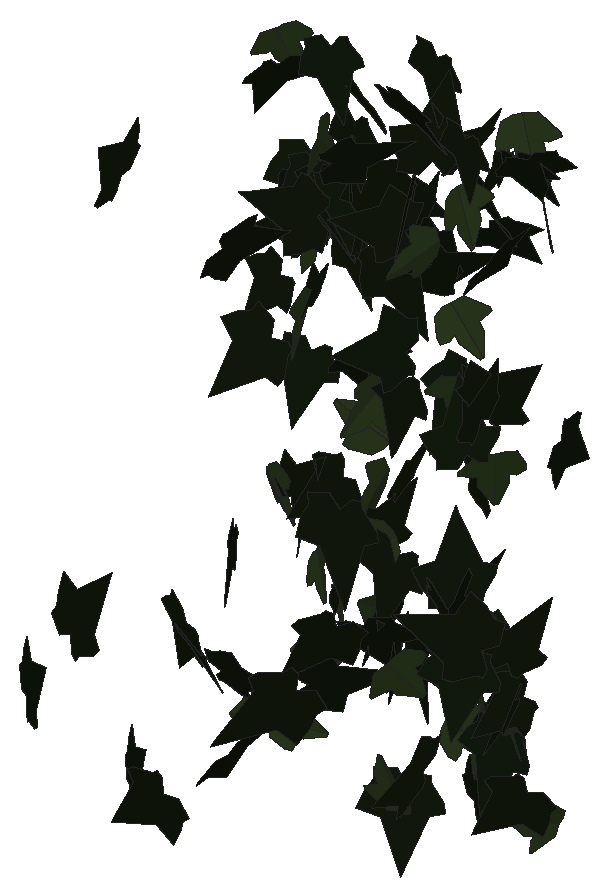
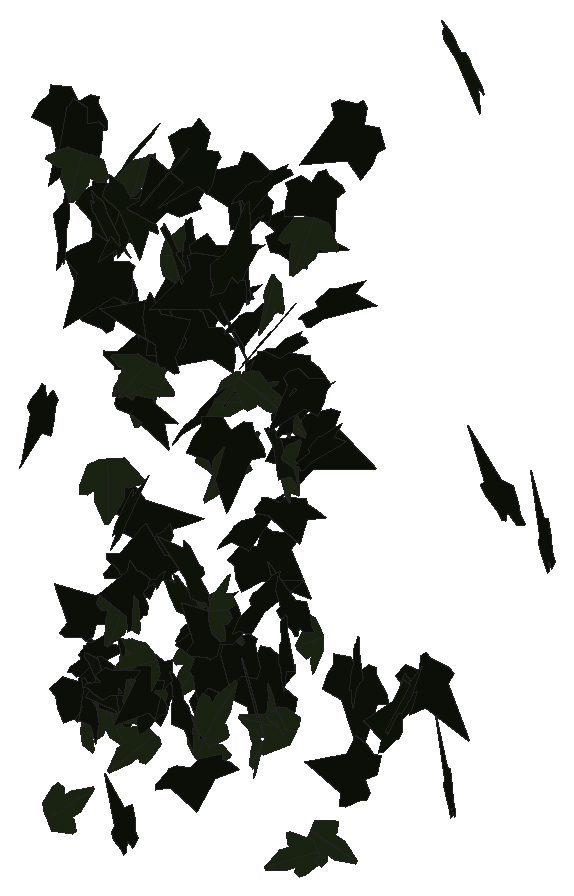
# SketchUp Ruby script. Lengths in inches.
U = 1.inch
M = Sketchup.active_model
def pt(a) = Geom::Point3d.new(a.map { |v| v * U })
def face(e, loops, mat)
  f = e.add_face(loops[0].map { |a| pt(a) })
  loops[1..].each { |l| e.add_face(l.map { |a| pt(a) }).erase! }
  f.material = f.back_material = mat if mat
  f
end
# faces: each face lists its corners as indices into pts; further lists are holes
def faces(e, pts, list, mat = nil) = list.each { |f| face(e, (f[0].is_a?(Array) ? f : [f]).map { |l| l.map { |i| pts[i] } }, mat) }
# xy, xz, yz: faces in a plane at the given z, y or x. An outline is a flat list of corners, or four numbers for a rectangle; further outlines are holes
def ring(l) = l.size == 4 ? [[l[0], l[1]], [l[2], l[1]], [l[2], l[3]], [l[0], l[3]]] : l.each_slice(2).to_a
def flat(e, list, mat, &to3) = list.each { |f| face(e, (f[0].is_a?(Array) ? f : [f]).map { |l| ring(l).map { |u, v| to3.(u, v) } }, mat) }
def xy(e, z, list, mat = nil) = flat(e, list, mat) { |x, y| [x, y, z] }
def xz(e, y, list, mat = nil) = flat(e, list, mat) { |x, z| [x, y, z] }
def yz(e, x, list, mat = nil) = flat(e, list, mat) { |y, z| [x, y, z] }
def lines(e, pts, list) = list.each { |a, b| e.add_line(pt(pts[a]), pt(pts[b])) }
# prism: a flat outline (further loops are holes) pulled along v
def prism(e, loops, v, mat = nil)
  f = face(e, loops, mat); d = Geom::Vector3d.new(v.map { |x| x * U })
  f.pushpull(f.normal.samedirection?(d) ? d.length : -d.length)
end
def box(e, o, s, mat = nil) = prism(e, [[o, [o[0] + s[0], o[1], o[2]], [o[0] + s[0], o[1] + s[1], o[2]], [o[0], o[1] + s[1], o[2]]]], [0, 0, s[2]], mat)
def at(x, y, z, deg = 0) = Geom::Transformation.translation(pt([x, y, z])) * Geom::Transformation.rotation(ORIGIN, Z_AXIS, deg.degrees)
def axes(o, x, y, z) = Geom::Transformation.new([*x, 0, *y, 0, *z, 0, *pt(o).to_a, 1])
def part(name) = M.definitions.add(name)
# library, detail: a bought-in or finely detailed component or shape, given as its bounding box
def library(name, o, s) = part(name).tap { |d| box(d.entities, o, s) }
def detail(e, o, s) = box(e.add_group.entities, o, s)
def put(e, d, t, mat = nil) = e.add_instance(d, t).tap { |i| i.material = mat if mat }
def group(e, t, mat = nil) = e.add_group.tap { |g| g.transformation = t; g.material = mat if mat }.entities
root = M.entities
M.materials.add("efeu1").color = [18, 25, 13]
M.materials.add("efeu2").color = [43, 57, 29]
c1 = part("ivyleaf_9")
p = [[1.54,2.16,1.25],[1.36,2.04,1.19],[-0.21,0.99,0.68],[-0.71,1.11,0.82],[-0.85,0.86,0.67],[-0.8,0.17,0.21],
  [-0.9,-0.01,0.1],[-0.67,-0.16,-0.02],[-0.08,-0.08,-0.05],[-0.03,-0.6,-0.4],[0.65,-0.88,-0.66],[0.83,-0.6,-0.49],
  [1.29,-0.42,-0.43],[1.8125,-0.07,-0.26],[1.21,0.44,0.15]]
faces(c1.entities,p,[[0,1,2,3,4,5,6,7,8,9,10,11,12,13,14]],"efeu1")
c2 = part("ivyleaf_10")
p = [[0,0.5,-0.03],[-0.0625,2.02,-0.43],[-0.19,2.01,-0.46],[-0.54,1.05,-0.29],[-0.52,0.625,-0.18],[-0.83,0.76,-0.28],
  [-1.16,0.64,-0.33],[-1.15,0.33,-0.24],[-0.77,-0.39,0.02],[-0.3,-0.51,0.16],[0.04,-0.48,0.23],[-0.02,2.01,-0.4375],
  [-0.06,2.01,-0.43],[0.04,-0.49,0.23],[0.67,-0.49,0.14],[1.38,0.36,-0.2],[1.375,0.51,-0.24],[0.81,0.65,-0.19],
  [0.62,0.59,-0.15],[0.6,1.09,-0.28],[0.5,1.23,-0.31]]
faces(c2.entities,p,[[0,1,2,3,4,5,6,7,8,9,10],[11,12,0,13,14,15,16,17,18,19,20]],"efeu2")
put(root,c1,axes([579.07,103.43,216.42],[-0.10825,0.38279,1.36931],[0.40428,-1.3083,0.39769],[1.36312,0.41843,-0.00921]))
put(root,c1,axes([580.27,105.16,219.3125],[-0.53768,0.6811,1.20334],[0.72427,-0.9611,0.86761],[1.17787,0.9019,0.01581]))
put(root,c1,axes([591.9,106.43,219.63],[-0.17555,0.07907,-1.48318],[-0.08289,-1.4917,-0.06971],[-1.48297,0.07402,0.17947]))
put(root,c1,axes([582.68,105.55,243.5625],[-0.49377,1.01434,0.96562],[-0.40798,0.87529,-1.12807],[-1.33973,-0.64039,-0.01237]))
put(root,c1,axes([583.03,108.125,210.53],[0.18388,0.19676,-1.31509],[-1.11192,-0.70534,-0.26101],[-0.72926,1.12506,0.06636]))
put(root,c1,axes([586.28,108.63,239.61],[-0.18844,0.58509,-1.22323],[-0.33091,1.1778,0.61434],[1.31496,0.38024,-0.02069]))
put(root,c1,axes([577.71,112.55,207.4],[-0.13971,0.48416,1.32584],[0.31161,-1.28886,0.50349],[1.37664,0.34088,0.02058]))
put(root,c1,axes([584.16,111.53,211.52],[-0.08745,1.35705,0.11136],[-0.02089,0.11024,-1.35979],[-1.36145,-0.08886,0.01371]))
put(root,c1,axes([584.93,113.43,232.34],[-0.69577,-0.9607,0.68415],[-0.35284,-0.5884,-1.18507],[1.12539,-0.77843,0.05142]))
put(root,c1,axes([594.11,112.95,213.47],[-1.09059,1.02972,0.10081],[-0.07995,0.06216,-1.49987],[-1.03155,-1.09347,0.00967]))
put(root,c1,axes([588.11,114.18,218.24],[0.01873,0.4628,-1.16576],[-0.19875,-1.15006,-0.45976],[-1.23842,0.19157,0.05615]))
put(root,c1,axes([577.84,116.36,213.89],[0.06024,-0.81055,1.02124],[0.21039,-1.00289,-0.80839],[1.28672,0.20192,0.08437]))
put(root,c1,axes([577.72,116.38,213.51],[0.76548,-0.83695,0.53558],[0.36072,-0.39589,-1.13422],[0.92586,0.84621,-0.00091]))
put(root,c1,axes([594.76,116.21,218.63],[-0.55565,0.09318,1.33177],[-1.30162,0.28283,-0.56287],[-0.29675,-1.41505,-0.02481]))
put(root,c1,axes([585.2,116.34,237.54],[-0.68854,-0.3639,-1.06199],[-0.83813,-0.66219,0.77031],[-0.74684,1.07862,0.11462]))
put(root,c1,axes([589.56,117.31,231.63],[-0.39556,-0.31287,1.22597],[-0.84982,-0.88592,-0.50029],[0.93738,-0.9352,0.06378]))
put(root,c1,axes([585.96,117.27,222.04],[0.02692,-1.50745,-0.09192],[0.02147,0.09231,-1.50751],[1.51009,0.02556,0.02307]))
put(root,c1,axes([593.33,117.1875,217],[-0.6421,-1.04679,-0.25794],[0.13029,0.22268,-1.22802],[1.0702,-0.65516,-0.00526]))
put(root,c2,axes([589.14,117.26,208.37],[-1.13639,0.18281,-0.28609],[-0.28191,0.04886,1.151],[0.1892,1.17083,-0.00336]))
put(root,c1,axes([594.77,116.34,230.57],[-0.27372,0.74434,1.24374],[-0.54005,1.12222,-0.79047],[-1.3451,-0.60203,0.06427]))
put(root,c2,axes([587.41,118.02,228.33],[0.19551,0.57216,-1.11063],[-0.29545,-1.07108,-0.6038],[-1.21391,0.35284,-0.03192]))
put(root,c1,axes([593.25,117.23,227.84],[-1.1164,-0.28305,0.34904],[0.33752,0.08897,1.15172],[-0.29669,1.1663,-0.00315]))
put(root,c1,axes([594.3125,117.54,230.48],[-0.3095,-0.0444,1.23471],[1.18697,-0.36398,0.28444],[0.34292,1.21976,0.12982]))
put(root,c1,axes([584.77,116.8125,213.03],[0.42859,0.84815,-1.03236],[0.37533,0.96409,0.94788],[1.28228,-0.56568,0.06761]))
put(root,c1,axes([585.76,117.18,240.09],[0.39198,0.87634,-0.84197],[0.22841,0.8158,0.95543],[1.19362,-0.4439,0.09367]))
put(root,c1,axes([578.46,118.33,210.85],[0.66587,-0.30071,0.89863],[0.83868,-0.32424,-0.72995],[0.44111,1.07041,0.03134]))
put(root,c2,axes([589.38,119.27,236.08],[0.0389,-0.29592,1.14624],[0.04383,-1.14571,-0.29727],[1.18301,0.05218,-0.02668]))
put(root,c1,axes([588.47,118.9375,208.11],[-0.47012,-1.23514,-0.35463],[0.09186,0.34435,-1.32111],[1.28175,-0.4777,-0.03539]))
put(root,c1,axes([595.4375,118.74,210.25],[0.1917,0.31235,-1.19576],[-0.68086,-0.98318,-0.36597],[-1.03142,0.70707,0.01934]))
put(root,c1,axes([578.39,119.07,217.43],[-0.19083,0.08645,-1.13172],[1.01876,-0.49288,-0.20943],[-0.50038,-1.03647,0.0052]))
put(root,c1,axes([590.61,118.32,218.99],[1.08634,-0.51397,-0.3688],[-0.32783,0.16939,-1.20173],[0.54102,1.13466,0.01235]))
put(root,c2,axes([591.96,118.54,239.77],[0.15481,1.18767,0.14534],[0.02303,0.14356,-1.19771],[-1.1963,0.15646,-0.00425]))
put(root,c2,axes([586.72,119.14,225.65],[0.46375,0.75342,0.87862],[-0.50905,-0.71729,0.88377],[1.03946,-0.68741,0.04081]))
put(root,c2,axes([588.19,118.4375,214.35],[-0.53396,-0.83901,-0.72053],[0.42714,0.58158,-0.99375],[1.02012,-0.68267,0.03895]))
put(root,c1,axes([581.1,118.87,242.69],[0.01534,0.92396,-0.61627],[-0.01956,-0.61601,-0.92406],[-1.11046,0.02362,0.00776]))
put(root,c1,axes([587.6875,119.6,236.26],[-0.36427,-0.16062,1.12111],[-1.03491,-0.43116,-0.39804],[0.46004,-1.09712,-0.00771]))
put(root,c1,axes([587.47,119.83,228.21],[0.03637,-1.2495,0.4438],[0.00807,-0.44375,-1.25002],[1.32595,0.03698,-0.00456]))
put(root,c1,axes([586.37,118.61,215.73],[1.06539,0.91543,-0.2444],[-0.18755,-0.15674,-1.40465],[-0.92874,1.08177,0.00329]))
put(root,c1,axes([593.56,118.49,237.02],[0.07385,1.31074,0.52223],[0.04213,0.52066,-1.31277],[-1.41032,0.08419,-0.01188]))
put(root,c1,axes([590.82,120.27,241.625],[0.20971,-1.05024,0.41894],[0.12344,-0.40227,-1.07025],[1.12395,0.24013,0.03938]))
put(root,c2,axes([582.64,119.11,212.43],[0.35874,0.20737,-1.07011],[0.88804,0.59767,0.41353],[0.63207,-0.9574,0.02636]))
put(root,c1,axes([592.63,120.625,211.32],[-0.31074,-1.22417,0.26123],[-0.06262,-0.25361,-1.263],[1.25017,-0.31699,0.00167]))
put(root,c1,axes([587.62,120.33,238.01],[-0.44358,0.2192,-1.02053],[0.90267,-0.47625,-0.49465],[-0.52414,-1.0057,0.01181]))
put(root,c1,axes([595.12,119.41,242.48],[0.65238,0.9812,-0.31935],[-0.18834,-0.25825,-1.17821],[-1.01453,0.67889,0.01337]))
put(root,c2,axes([590.69,119.98,229.16],[-0.92639,-0.66734,-0.04645],[0.03859,0.0259,-1.14173],[0.66784,-0.92719,0.00154]))
put(root,c1,axes([590.79,119.87,218.72],[-1.14982,-0.33328,0.46317],[0.46405,0.06015,1.1953],[-0.33206,1.23814,0.0666]))
put(root,c1,axes([587.1,119.74,242.83],[1.34869,-0.02993,-0.15899],[-0.15879,0.01054,-1.34901],[0.03095,1.35799,0.00697]))
put(root,c1,axes([593.375,120.45,213.49],[-0.90631,0.48453,-0.55537],[0.45776,-0.31982,-1.02605],[-0.57763,-1.01368,0.05826]))
put(root,c1,axes([593.3125,121.09,213.47],[-0.42341,-0.74785,0.71431],[-0.37697,-0.60715,-0.85911],[0.96303,-0.56647,-0.02223]))
put(root,c1,axes([586.23,121.12,218.2],[-0.19454,-1.21348,0.33962],[-0.05976,-0.33437,-1.22896],[1.25869,-0.20343,-0.00586]))
put(root,c2,axes([579.35,120.55,208.27],[-0.33738,-0.11776,0.98164],[-0.88497,-0.42647,-0.35531],[0.4408,-0.94634,0.03798]))
put(root,c1,axes([583.43,121.01,237.27],[-0.16567,0.42932,1.36524],[0.20507,-1.35305,0.45038],[1.41638,0.24612,0.09448]))
put(root,c1,axes([583.85,120.98,239.71],[0.22097,-1.07032,0.18904],[0.03184,-0.18645,-1.09287],[1.08642,0.22316,-0.00642]))
put(root,c1,axes([594.11,120.02,241.94],[1.10862,0.29189,-0.22986],[-0.22128,-0.06232,-1.14639],[-0.29844,1.13048,-0.00385]))
put(root,c1,axes([582.63,120.83,243.23],[0.04728,-1.1338,-0.26417],[0.0458,0.266,-1.13343],[1.16327,0.03561,0.05536]))
put(root,c1,axes([580.5625,120.65,219.64],[-0.35822,0.39749,1.00042],[0.65931,-0.75246,0.53505],[0.85097,0.75031,0.00658]))
put(root,c1,axes([585.98,121.03,216.02],[-0.40139,0.48456,-0.93814],[0.62262,-0.70197,-0.62897],[-0.85279,-0.74058,-0.01765]))
put(root,c1,axes([586.14,120.65,233.85],[-0.45288,-0.44446,-1.25416],[1.0157,0.74035,-0.62914],[0.85955,-1.10901,0.08264]))
put(root,c2,axes([591.91,121.05,211.23],[-0.20329,-1.07425,0.46882],[-0.04198,-0.46884,-1.0925],[1.17135,-0.20324,0.04221]))
put(root,c1,axes([591.41,119.6875,212.81],[0.00703,0.47244,1.11694],[-0.04457,1.11631,-0.47189],[-1.21193,-0.03831,0.02384]))
put(root,c1,axes([586.86,119.83,212.54],[-0.00786,-0.02968,1.24119],[0.14201,1.23305,0.03039],[-1.2334,0.14216,-0.00441]))
put(root,c1,axes([579.03,121.54,229.99],[-0.30255,-0.81607,0.64489],[-0.23167,-0.60188,-0.87033],[1.014,-0.38101,-0.00643]))
put(root,c1,axes([590.06,121.22,228.67],[-1.16405,-0.41683,-0.3484],[0.32775,0.11817,-1.23643],[0.43326,-1.20931,-0.00073]))
put(root,c1,axes([582.33,121.85,220.54],[0.28135,-0.59823,-1.15429],[0.50544,-1.03777,0.66104],[-1.19783,-0.57842,0.00781]))
put(root,c1,axes([588.45,120.09,237.07],[-0.16861,0.63322,0.93226],[-0.3138,0.87898,-0.65379],[-1.08241,-0.35346,0.04432]))
put(root,c2,axes([591.23,120.73,217.08],[-1.17774,0.25113,-0.20413],[0.20259,-0.0287,-1.20414],[-0.25238,-1.19496,-0.01398]))
put(root,c1,axes([590.82,119.83,217.4],[0.06754,0.20457,1.36192],[0.52321,1.25751,-0.21483],[-1.27394,0.52731,-0.01602]))
put(root,c2,axes([579.01,121.27,219.69],[-0.59955,0.4755,-0.89578],[0.68796,-0.57389,-0.76508],[-0.74514,-0.91244,0.01439]))
put(root,c1,axes([582.77,121.29,236.16],[0.00295,-1.058,-0.30134],[-0.00093,0.30134,-1.058],[1.10008,0.00309,-0.00009]))
put(root,c1,axes([584.78,120.54,228.53],[0.40309,1.18402,-0.32712],[-0.09964,-0.31163,-1.25074],[-1.22433,0.41518,-0.00591]))
put(root,c2,axes([591.42,120.29,213.67],[0.30909,0.1469,-1.17444],[-0.65574,1.03176,-0.04353],[0.98533,0.64055,0.33944]))
put(root,c2,axes([585.56,121.03,218.89],[0.65178,-0.1511,-0.89316],[-0.86433,0.22558,-0.6689],[0.27112,1.08243,0.01472]))
put(root,c1,axes([580.74,121.63,226.54],[-0.83532,-0.7343,-0.38515],[0.28887,0.25473,-1.11218],[0.77723,-0.88386,-0.00056]))
put(root,c1,axes([588.44,120.86,239.71],[-0.85134,-0.53973,0.95737],[0.86353,0.4206,1.00502],[-0.67983,1.21014,0.07768]))
put(root,c1,axes([592.92,120.76,215.43],[-0.37995,-0.22674,1.07804],[0.98111,0.44898,0.44022],[-0.50101,1.05117,0.04451]))
put(root,c2,axes([580.27,121.88,228.88],[0.42187,-0.93876,0.71655],[0.43374,-0.58455,-1.0212],[1.09844,0.59136,0.12804]))
put(root,c1,axes([581.47,121.5,235.76],[0.64766,-1.1767,-0.22257],[-0.03994,0.23166,-1.34103],[1.1969,0.64446,0.07568]))
put(root,c1,axes([584.57,120.66,234.27],[-0.06526,0.41749,1.02702],[-0.45521,0.92798,-0.40616],[-1.01087,-0.44484,0.1166]))
put(root,c1,axes([588.59,121.38,213.3],[1.14859,-0.56147,0.553],[0.49667,-0.24318,-1.27847],[0.61186,1.25137,-0.00032]))
put(root,c1,axes([587.89,120.8,233.53],[0.41685,0.09656,1.227],[1.18615,0.31422,-0.42771],[-0.32848,1.2572,0.01266]))
put(root,c1,axes([586.67,121.86,213.76],[-0.40361,-0.0541,-1.27166],[1.27277,-0.02724,-0.4028],[-0.00962,-1.33389,0.0598]))
put(root,c2,axes([589.08,121.64,214.98],[-0.64518,0.19285,-0.96428],[0.91252,-0.31243,-0.67303],[-0.36652,-1.11735,0.02176]))
put(root,c1,axes([591.52,120.58,212.25],[-0.67348,0.8523,-0.68627],[-0.41819,0.54418,1.08624],[1.01118,0.79272,-0.00784]))
put(root,c2,axes([579.73,121.02,207.46],[0.18962,0.2276,0.98077],[0.55608,0.80831,-0.29509],[-0.83934,0.58694,0.02607]))
put(root,c1,axes([584.85,120.93,237.19],[0.11276,0.04854,-1.35483],[0.52297,1.25272,0.08841],[1.25077,-0.52816,0.08517]))
put(root,c1,axes([582.74,122,232.82],[0.47582,-0.99644,-0.07122],[-0.02712,0.06597,-1.10421],[0.99861,0.47658,0.00395]))
put(root,c2,axes([591.37,121.74,224.63],[-0.78246,-0.96482,-0.0071],[0.00086,0.00844,-1.24222],[0.96485,-0.78245,-0.00465]))
put(root,c1,axes([590.01,121.62,238.91],[1.0879,-0.68166,-0.25782],[-0.20613,0.15652,-1.28361],[0.69903,1.10702,0.02273]))
put(root,c2,axes([584.7,121.125,227.11],[-0.03954,-0.5253,-0.98037],[0.02866,0.98018,-0.52636],[1.11187,-0.04395,-0.0213]))
put(root,c1,axes([580.0625,122.47,219.62],[-0.41463,0.22846,-1.176],[1.0667,-0.49602,-0.47246],[-0.54528,-1.14406,-0.03]))
put(root,c2,axes([581.49,121.37,237.98],[0.14706,-0.7576,-0.84923],[0.00288,0.85653,-0.76361],[1.13804,0.09573,0.11168]))
put(root,c2,axes([580.61,122.29,215.56],[0.55786,-0.22346,0.80115],[0.7449,-0.29489,-0.60095],[0.36999,0.93063,0.00195]))
put(root,c2,axes([578.96,121.79,242.29],[-0.7666,-0.75984,-0.39655],[0.28393,0.27685,-1.07936],[0.8087,-0.81749,0.00305]))
put(root,c2,axes([589.37,121.375,210.42],[0.26974,0.62154,0.87728],[0.33047,0.81275,-0.67743],[-1.02309,0.4264,0.01248]))
put(root,c2,axes([592.73,121.65,210.25],[-0.594,0.69191,-0.71844],[-0.47156,0.54203,0.9119],[0.87893,0.75841,0.00371]))
put(root,c2,axes([588.94,121.9375,231.3],[0.7417,0.55782,0.63925],[0.51683,0.37629,-0.92802],[-0.67283,0.90398,-0.00817]))
put(root,c2,axes([584.09,123.08,213.84],[-0.13627,-0.64275,-1.07106],[-0.26001,-1.03921,0.65672],[-1.22175,0.29285,-0.0203]))
put(root,c1,axes([579.51,123.05,232.16],[-0.23575,-0.18916,1.08119],[-0.65428,-0.86368,-0.29377],[0.88129,-0.69181,0.07113]))
put(root,c1,axes([580.83,121.44,229.27],[-0.00143,0.58859,0.92022],[-0.22887,0.89963,-0.57578],[-1.06811,-0.19356,0.12214]))
put(root,c1,axes([582.69,121.41,215.08],[0.0059,0.25888,1.28019],[-0.30397,1.24533,-0.25043],[-1.27024,-0.29681,0.06587]))
put(root,c2,axes([580.45,121.89,232.07],[0.22033,-0.17233,-1.04982],[-0.84286,0.6259,-0.27963],[0.64916,0.87115,-0.00676]))
put(root,c1,axes([580.37,122.59,235.59],[0.01246,-1.15684,-0.28258],[0.00521,0.28264,-1.15688],[1.19084,0.01086,0.00801]))
put(root,c2,axes([583.55,123.16,220.35],[0.15471,-0.43656,1.18067],[0.54299,-1.05004,-0.45942],[1.13566,0.56153,0.05882]))
put(root,c2,axes([588.98,121.84,212.49],[0.66751,0.77562,-0.50549],[0.29664,0.41114,1.02257],[0.87699,-0.72942,0.03886]))
put(root,c1,axes([595.28,121.66,227.11],[0.12146,-0.14507,-1.19635],[-0.86522,0.82649,-0.18806],[0.83887,0.87345,-0.02075]))
put(root,c1,axes([588.55,121.5,213.95],[-0.1594,0.30396,-1.08576],[-0.45146,0.98761,0.34276],[1.03317,0.47845,-0.01774]))
put(root,c1,axes([590.06,122.5625,222.29],[0.16659,-1.0426,0.66961],[-0.10748,0.66093,1.05582],[-1.23444,-0.19825,-0.00156]))
put(root,c1,axes([591.51,122.79,212.39],[-0.25,0.02469,-1.05952],[1.05919,-0.03135,-0.25066],[-0.03619,-1.08816,-0.01682]))
put(root,c2,axes([593.27,123.29,205.96],[-0.29936,-0.21025,-0.99804],[-0.56257,-0.83358,0.34434],[-0.85077,0.62518,0.12349]))
put(root,c1,axes([589.18,123.03,205.94],[-0.09001,0.12812,1.13543],[0.5463,-0.99552,0.15564],[1.00358,0.5534,0.01711]))
put(root,c1,axes([584.19,122.17,218.06],[-0.28685,-0.30355,1.04085],[0.93189,0.48128,0.39718],[-0.55417,0.96645,0.12913]))
put(root,c1,axes([586.7,123.35,242.99],[0.18216,-1.10973,0.43678],[0.11189,-0.42399,-1.12391],[1.18733,0.21021,0.03891]))
put(root,c1,axes([587.88,122.32,233.18],[0.18576,-0.22916,1.33655],[-0.79515,1.07437,0.29472],[-1.09846,-0.81646,0.01268]))
put(root,c1,axes([589.8,121.87,240.12],[-0.17635,1.14308,0.65088],[-0.35896,0.58996,-1.13335],[-1.26548,-0.32664,0.23078]))
put(root,c1,axes([591.01,122.93,239.8],[-0.90207,0.44261,-0.47873],[0.40983,-0.25067,-1.004],[-0.50707,-0.98999,0.04018]))
put(root,c1,axes([590.93,122.02,236.34],[1.03181,0.76814,0.0973],[0.06746,0.07232,-1.28622],[-0.77133,1.03386,0.01767]))
put(root,c1,axes([585.49,122.13,221.11],[-0.46526,1.15258,0.11734],[0.02786,-0.11528,1.24282],[1.1582,0.46577,0.01725]))
put(root,c1,axes([582.29,123.51,239.51],[1.09483,-0.72481,-0.33774],[0.28628,-0.17939,1.31299],[-0.74664,-1.13161,0.00818]))
put(root,c1,axes([578.73,122.02,234.22],[0.00501,-0.06713,-1.08285],[-0.36203,1.02069,-0.06495],[1.02274,0.36164,-0.01769]))
put(root,c1,axes([590.28,123.43,214.24],[-0.90489,-0.49147,0.48713],[-0.42252,-0.24265,-1.02969],[0.54801,-0.99862,0.01046]))
put(root,c2,axes([581.2,123,213.67],[-0.53491,0.59356,-0.55869],[0.31466,-0.46609,-0.79645],[-0.75196,-0.61728,0.06415]))
put(root,c2,axes([592.22,122.67,241.79],[1.04179,0.53941,0.32806],[0.23748,0.2517,-1.16798],[-0.58498,1.06283,0.1101]))
put(root,c1,axes([579.61,123.21,235.53],[-0.75083,-0.89142,-0.58993],[0.38657,0.44569,-1.16547],[0.9966,-0.84446,0.00762]))
put(root,c1,axes([592.56,123.5,238.3],[0.265,-0.18663,-1.27978],[1.24827,-0.30487,0.30293],[-0.33836,-1.27088,0.11527]))
put(root,c2,axes([581.57,122.98,233.43],[0.69075,-0.00426,-0.99408],[-0.9938,0.02619,-0.69067],[0.02394,1.21023,0.01145]))
